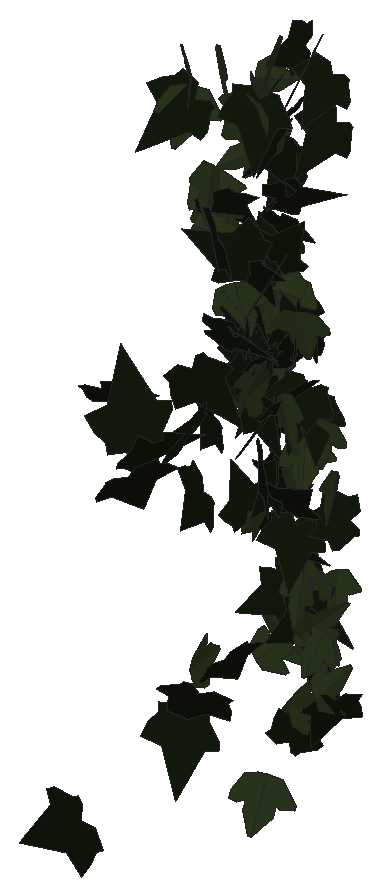
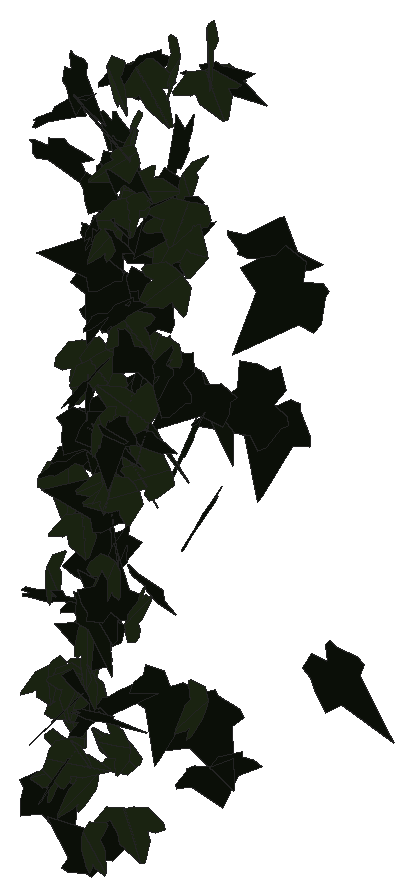
# SketchUp Ruby script. Lengths in inches.
U = 1.inch
M = Sketchup.active_model
def pt(a) = Geom::Point3d.new(a.map { |v| v * U })
def face(e, loops, mat)
  f = e.add_face(loops[0].map { |a| pt(a) })
  loops[1..].each { |l| e.add_face(l.map { |a| pt(a) }).erase! }
  f.material = f.back_material = mat if mat
  f
end
# faces: each face lists its corners as indices into pts; further lists are holes
def faces(e, pts, list, mat = nil) = list.each { |f| face(e, (f[0].is_a?(Array) ? f : [f]).map { |l| l.map { |i| pts[i] } }, mat) }
# xy, xz, yz: faces in a plane at the given z, y or x. An outline is a flat list of corners, or four numbers for a rectangle; further outlines are holes
def ring(l) = l.size == 4 ? [[l[0], l[1]], [l[2], l[1]], [l[2], l[3]], [l[0], l[3]]] : l.each_slice(2).to_a
def flat(e, list, mat, &to3) = list.each { |f| face(e, (f[0].is_a?(Array) ? f : [f]).map { |l| ring(l).map { |u, v| to3.(u, v) } }, mat) }
def xy(e, z, list, mat = nil) = flat(e, list, mat) { |x, y| [x, y, z] }
def xz(e, y, list, mat = nil) = flat(e, list, mat) { |x, z| [x, y, z] }
def yz(e, x, list, mat = nil) = flat(e, list, mat) { |y, z| [x, y, z] }
def lines(e, pts, list) = list.each { |a, b| e.add_line(pt(pts[a]), pt(pts[b])) }
# prism: a flat outline (further loops are holes) pulled along v
def prism(e, loops, v, mat = nil)
  f = face(e, loops, mat); d = Geom::Vector3d.new(v.map { |x| x * U })
  f.pushpull(f.normal.samedirection?(d) ? d.length : -d.length)
end
def box(e, o, s, mat = nil) = prism(e, [[o, [o[0] + s[0], o[1], o[2]], [o[0] + s[0], o[1] + s[1], o[2]], [o[0], o[1] + s[1], o[2]]]], [0, 0, s[2]], mat)
def at(x, y, z, deg = 0) = Geom::Transformation.translation(pt([x, y, z])) * Geom::Transformation.rotation(ORIGIN, Z_AXIS, deg.degrees)
def axes(o, x, y, z) = Geom::Transformation.new([*x, 0, *y, 0, *z, 0, *pt(o).to_a, 1])
def part(name) = M.definitions.add(name)
# library, detail: a bought-in or finely detailed component or shape, given as its bounding box
def library(name, o, s) = part(name).tap { |d| box(d.entities, o, s) }
def detail(e, o, s) = box(e.add_group.entities, o, s)
def put(e, d, t, mat = nil) = e.add_instance(d, t).tap { |i| i.material = mat if mat }
def group(e, t, mat = nil) = e.add_group.tap { |g| g.transformation = t; g.material = mat if mat }.entities
root = M.entities
M.materials.add("efeu1").color = [18, 25, 13]
M.materials.add("efeu2").color = [43, 57, 29]
c1 = part("ivyleaf_9")
p = [[1.54,2.16,1.25],[1.36,2.04,1.19],[-0.21,0.99,0.68],[-0.71,1.11,0.82],[-0.85,0.86,0.67],[-0.8,0.17,0.21],
  [-0.9,-0.01,0.1],[-0.67,-0.16,-0.02],[-0.08,-0.08,-0.05],[-0.03,-0.6,-0.4],[0.65,-0.88,-0.66],[0.83,-0.6,-0.49],
  [1.29,-0.42,-0.43],[1.8125,-0.07,-0.26],[1.21,0.44,0.15]]
faces(c1.entities,p,[[0,1,2,3,4,5,6,7,8,9,10,11,12,13,14]],"efeu1")
c2 = part("ivyleaf_10")
p = [[0,0.5,-0.03],[-0.0625,2.02,-0.43],[-0.19,2.01,-0.46],[-0.54,1.05,-0.29],[-0.52,0.625,-0.18],[-0.83,0.76,-0.28],
  [-1.16,0.64,-0.33],[-1.15,0.33,-0.24],[-0.77,-0.39,0.02],[-0.3,-0.51,0.16],[0.04,-0.48,0.23],[-0.02,2.01,-0.4375],
  [-0.06,2.01,-0.43],[0.04,-0.49,0.23],[0.67,-0.49,0.14],[1.38,0.36,-0.2],[1.375,0.51,-0.24],[0.81,0.65,-0.19],
  [0.62,0.59,-0.15],[0.6,1.09,-0.28],[0.5,1.23,-0.31]]
faces(c2.entities,p,[[0,1,2,3,4,5,6,7,8,9,10],[11,12,0,13,14,15,16,17,18,19,20]],"efeu2")
put(root,c1,axes([507.44,115.02,209.63],[0.08997,-0.01027,-1.35378],[-1.25282,-0.59245,-0.07234],[-0.63793,1.16206,-0.04885]))
put(root,c1,axes([508.96,117.2,228.68],[-1.34114,-0.18158,0.15582],[0.16312,0.00251,1.30505],[-0.19503,1.2508,0.02]))
put(root,c1,axes([506.04,118.68,229.07],[1.25105,0.55078,0.11177],[0.01308,0.22191,-1.31853],[-0.60591,1.142,0.20231]))
put(root,c1,axes([506.1,120.25,223.99],[0.4219,1.17908,-0.04223],[-0.01786,-0.0373,-1.29179],[-1.27404,0.39097,0.00412]))
put(root,c1,axes([505.62,121.05,224.76],[0.5397,0.46317,1.00584],[0.78935,0.63368,-0.70835],[-0.84746,0.88519,-0.01921]))
put(root,c1,axes([508.71,123.16,235.53],[0.12597,-0.53017,1.05207],[0.21043,-0.99273,-0.56445],[1.2154,0.22683,-0.01132]))
put(root,c1,axes([507.36,122.56,225.4],[-0.38072,1.00645,0.44945],[-0.22304,0.38477,-1.10713],[-1.16171,-0.40371,0.06527]))
put(root,c1,axes([506.3,124.34,241.09],[-1.0487,-0.46693,0.20114],[-0.15215,-0.15224,-1.11784],[0.5242,-0.97832,0.07795]))
put(root,c1,axes([505.75,124.66,209.75],[-0.47823,-1.02183,-0.19653],[0.05573,0.18354,-1.1579],[1.12091,-0.44508,-0.02628]))
put(root,c1,axes([506.83,124.12,211.76],[0.2588,0.74456,-0.84826],[-0.66024,-0.60564,-0.76177],[-0.9933,0.59656,0.28533]))
put(root,c2,axes([506.02,124.44,241.03],[0.87954,0.69197,-0.27208],[-0.21436,-0.17045,-1.11142],[-0.76967,0.83823,-0.00139]))
put(root,c1,axes([505.96,125.45,220.92],[-0.08084,-0.67951,0.85136],[-0.06969,-0.81623,-0.71076],[1.14689,-0.09749,0.01682]))
put(root,c2,axes([506.28,124.08,242.47],[0.41246,-0.38741,-0.98564],[-0.40224,0.88964,-0.53431],[1.03001,0.50257,0.18603]))
put(root,c2,axes([506.31,125.57,236.73],[-0.01653,-0.79261,0.64627],[0.55281,-0.54136,-0.70502],[0.9368,0.30548,0.42744]))
put(root,c1,axes([505.97,124.94,227.1875],[-0.18311,-0.32095,-1.01861],[0.50476,0.86074,-0.37748],[0.99211,-0.49716,0.00405]))
put(root,c1,axes([509.87,124.8,223.77],[0.33491,-0.07966,-1.14204],[-1.15928,0.23192,-0.33275],[0.26453,1.11724,-0.01235]))
put(root,c1,axes([506.06,126.04,224.5],[0.01792,-0.5786,0.86533],[0.03632,-0.83139,-0.60196],[1.09393,0.03708,0.00581]))
put(root,c1,axes([508.85,125.83,241.18],[-0.33776,-1.00359,-0.16345],[0.06068,0.1471,-1.09319],[1.09541,-0.3176,0.01016]))
put(root,c2,axes([508.54,125.55,240.79],[0.95987,-0.02679,-0.65752],[-0.65396,0.2806,-0.89763],[0.1985,1.05399,0.22226]))
put(root,c1,axes([507.81,126.17,232.83],[-0.03618,0.02535,1.09537],[-1.0952,-0.28653,-0.02637],[0.30855,-1.01407,0.03484]))
put(root,c2,axes([506.14,124.98,212.54],[0.01911,-0.0001,1.0335],[-0.43086,0.9103,0.00748],[-0.98297,-0.39901,0.01681]))
put(root,c2,axes([506.44,126.13,242.39],[-0.44859,0.65457,-0.70694],[0.37319,-0.58561,-0.80606],[-0.94839,-0.54005,0.0172]))
put(root,c2,axes([508.87,126.05,207.02],[1.0544,0.46078,-0.17471],[-0.17122,-0.05763,-1.12264],[-0.50125,0.98896,0.01598]))
put(root,c1,axes([507.33,125.39,213.08],[0.21982,1.0348,0.13224],[0.03533,0.12316,-1.09678],[-1.12544,0.20598,-0.0086]))
put(root,c1,axes([506.67,125.5,235.77],[0.86317,0.60789,0.11341],[0.08365,0.07827,-1.04418],[-0.66173,0.80283,0.01593]))
put(root,c2,axes([505.88,125.79,233.96],[-0.18129,-0.19362,-0.93562],[0.93953,0.26479,-0.22808],[0.32406,-0.87601,0.13786]))
put(root,c2,axes([506.23,126.15,234.88],[-0.93752,-0.3321,-0.36595],[0.34974,0.13822,-0.96652],[0.38825,-0.92643,-0.01302]))
put(root,c2,axes([505.82,126.24,235.84],[0.70934,0.69682,0.28521],[0.18068,0.21902,-0.99546],[-0.78831,0.67721,0.02848]))
put(root,c1,axes([509.09,126.6875,238.78],[-0.71579,0.80943,-0.05822],[0.04619,-0.03733,-1.08796],[-0.87506,-0.66408,-0.00981]))
put(root,c1,axes([505.65,126.8,228.3],[0.84135,-0.1688,0.59998],[0.61407,-0.09942,-0.82876],[0.21059,0.96427,0.01958]))
put(root,c1,axes([508.46,127.58,225.33],[-0.73678,0.42455,-0.66813],[0.42124,-0.54953,-0.80843],[-0.71707,-0.75904,0.21158]))
put(root,c2,axes([505.71,127.2,233.07],[-0.76525,-0.01167,-0.63167],[0.65559,-0.04987,-0.73549],[-0.0255,-0.93192,0.04727]))
put(root,c2,axes([507.19,127.71,226.29],[0.13801,-0.90063,0.35682],[0.02235,-0.34345,-0.94565],[1.04063,0.12682,-0.02701]))
put(root,c2,axes([508.88,127.62,225.26],[-0.76283,0.4005,-0.6504],[0.42127,-0.53437,-0.81406],[-0.6825,-0.77747,0.22448]))
put(root,c2,axes([506.88,128.1,237.125],[-0.19217,-0.08229,0.95261],[-0.22671,-0.9047,-0.12693],[0.96701,-0.22846,0.15955]))
put(root,c1,axes([506.95,127.05,231.89],[1.0143,0.44026,-0.21916],[-0.21302,-0.07567,-1.07862],[-0.48218,0.95954,0.0155]))
put(root,c2,axes([506.32,127.36,230.08],[0.89877,0.3439,0.34767],[0.26468,0.27058,-0.92396],[-0.44524,0.85504,0.15256]))
put(root,c2,axes([507.61,127.02,225.68],[0.13359,0.025,1.04989],[-0.49921,0.90565,0.03557],[-0.96964,-0.46282,0.12633]))
put(root,c1,axes([506.86,127.71,226.78],[-0.91082,0.6213,0.08213],[-0.06815,0.04749,-1.0894],[-0.67296,-0.84571,-0.00084]))
put(root,c1,axes([505.74,127.71,229.44],[0.97194,-0.39811,-0.01221],[-0.00942,0.0093,-1.02342],[0.43004,0.89998,0.00518]))
put(root,c1,axes([507.88,128.03,231.24],[-0.68619,0.60856,-0.55886],[0.36228,-0.4246,-0.91258],[-0.79846,-0.71565,0.06621]))
put(root,c1,axes([506.02,127.82,228.96],[0.67776,-0.69422,-0.18064],[0.03874,0.26125,-0.95113],[0.7719,0.59644,0.20635]))
put(root,c1,axes([507.35,128.84,220.66],[0.11805,-0.25377,-0.92422],[0.6525,-0.65756,0.27257],[-0.75533,-0.60771,0.09102]))
put(root,c2,axes([509.03,128.38,216.18],[0.9726,-0.36527,0.1887],[0.18449,-0.06158,-1.01066],[0.39998,0.91658,0.0073]))
put(root,c2,axes([507.68,128.48,242.33],[0.44859,-0.80434,0.22061],[0.0845,-0.19827,-0.94121],[0.8944,0.42215,-0.02172]))
put(root,c1,axes([508.1,128.42,219.93],[0.9963,0.16764,-0.22796],[0.23199,0.04388,0.9751],[0.18709,-0.94717,0.00483]))
put(root,c1,axes([506.52,127.92,219.23],[-0.84481,0.10836,-0.41463],[-0.42477,0.06608,0.82122],[0.13663,0.87549,-0.01066]))
put(root,c1,axes([508.7,127.79,225.5],[0.07501,1.0197,0.12341],[-0.04429,0.12159,-1.06173],[-1.10782,0.06418,0.05081]))
put(root,c1,axes([506.59,128.35,224.45],[0.46268,-0.77355,-0.44589],[-0.22098,0.37678,-0.91963],[0.92926,0.47475,0.00332]))
put(root,c2,axes([507.21,127.91,239.12],[-0.45445,0.66627,0.7094],[-0.44787,0.5435,-0.81817],[-0.92731,-0.58902,0.0475]))
put(root,c1,axes([507.01,128.71,225.55],[-0.97848,0.22479,-0.43446],[0.43938,-0.09503,-0.97079],[-0.26352,-0.99314,-0.00545]))
put(root,c1,axes([507.68,128.39,227.42],[-0.76916,0.71124,-0.03933],[0.0289,-0.02672,-1.04678],[-0.76868,-0.71269,-0.00001]))
put(root,c1,axes([506.18,128.85,226.64],[-0.91785,-0.30376,-0.2525],[0.25534,0.05967,-0.93832],[0.33344,-0.88184,0.02349]))
put(root,c1,axes([506.66,128.03,228.79],[0.28397,-0.16805,-0.94821],[-0.81398,0.51313,-0.32441],[0.58307,0.79819,0.00892]))
put(root,c1,axes([506.85,127.7,226.29],[0.45607,0.49532,0.79481],[0.35402,0.70327,-0.66241],[-0.91765,0.51749,0.13946]))
put(root,c2,axes([507.16,127.86,239.62],[0.1305,0.07209,-1.06108],[-0.38997,0.96423,0.02638],[1.03352,0.35472,0.14394]))
put(root,c1,axes([508.37,129,218.44],[-0.45789,-0.83346,-0.21433],[0.15488,0.15787,-0.97082],[0.91422,-0.44419,0.05712]))
put(root,c2,axes([506.05,129.31,218.43],[-0.155,-0.02636,0.99927],[0.49477,-0.85593,0.04674],[0.91261,0.45956,0.14438]))
put(root,c2,axes([508.96,128.5625,229.17],[-1.0021,-0.3163,-0.06562],[0.07047,0.00409,-1.01935],[0.34113,-0.93,0.01784]))
put(root,c1,axes([508.83,129.17,225.34],[-0.51747,-0.86558,-0.0449],[0.02622,0.0359,-1.02891],[0.93562,-0.47973,0.004]))
put(root,c1,axes([505.81,129.24,226.01],[-0.21173,0.05111,0.8772],[-0.09857,-0.86208,0.03227],[0.90727,-0.08174,0.20822]))
put(root,c1,axes([507.35,128.89,231.55],[-0.437,-0.09411,0.84024],[0.81337,-0.38421,0.34572],[0.33183,0.81783,0.25911]))
put(root,c2,axes([509.58,128.99,213.24],[0.9711,-0.11072,-0.22862],[-0.22949,0.07106,-0.94112],[0.13418,0.92292,0.04504]))
put(root,c1,axes([509.14,129.23,242.3],[-0.64052,0.47663,-0.63476],[0.48774,-0.41164,-0.7907],[-0.67941,-0.74486,0.03079]))
put(root,c2,axes([506.67,128.9,211.65],[0.59089,0.00255,-0.68115],[0.7065,0.03982,0.56849],[0.03477,-0.85248,0.02452]))
put(root,c1,axes([509.14,129.5,224.7],[-0.21326,-0.93064,-0.05289],[0.13034,0.02601,-0.98247],[0.99812,-0.20224,0.117]))
put(root,c2,axes([507.57,129.55,229.56],[0.24724,0.30911,0.94114],[-0.55467,-0.74519,0.39984],[0.8712,-0.56216,-0.01252]))
put(root,c2,axes([505.38,128.6,225.08],[0.28419,0.25641,0.99116],[0.64866,0.74106,-0.37982],[-0.84579,0.65449,0.04174]))
put(root,c2,axes([506.21,129.375,231.81],[0.43438,0.61703,-0.47359],[-0.31367,-0.35335,-0.76471],[-0.76653,0.49425,0.04454]))
put(root,c2,axes([509.54,129.16,223.79],[-1.04599,-0.16051,0.06807],[-0.04444,-0.14796,-1.01072],[0.18185,-0.95938,0.14449]))
put(root,c1,axes([507.67,129.84,235.69],[-0.21757,-0.07069,0.89172],[-0.37315,-0.79984,-0.153],[0.85094,-0.36881,0.1609]))
put(root,c1,axes([508.15,129.95,213.35],[-0.26613,-0.45234,0.77032],[-0.35548,-0.66374,-0.53545],[0.8673,-0.41085,0.01691]))
put(root,c1,axes([507.03,129.88,214.32],[-0.48449,-0.36942,0.66604],[-0.40699,-0.53023,-0.59262],[0.68697,-0.57467,0.11863]))
put(root,c1,axes([509.91,129.67,238.81],[-0.98814,-0.32416,-0.09378],[0.08423,0.04982,-1.00927],[0.35349,-0.91803,-0.02165]))
put(root,c1,axes([507.85,129.88,228.7],[-0.06546,-0.0725,-0.91372],[0.85551,-0.39096,-0.02328],[-0.41783,-0.78913,0.09548]))
put(root,c1,axes([507.45,129.0625,233.5],[0.88337,0.27108,-0.42302],[-0.42251,-0.11234,-0.89602],[-0.31651,0.90656,0.01546]))
put(root,c1,axes([506.78,129.82,232.4],[-0.26718,-0.85675,-0.04992],[0.01475,0.04602,-0.92742],[0.92662,-0.24776,0.00037]))
put(root,c2,axes([509.18,129.02,213.59],[-0.15302,-0.66704,0.7175],[0.32919,0.62999,0.69858],[-0.98274,0.31489,0.12228]))
put(root,c1,axes([506.91,129.125,218.16],[0.30495,0.81151,0.05275],[-0.06369,-0.03311,0.89239],[0.87583,-0.28496,0.04653]))
put(root,c2,axes([508.8,128.6875,209.79],[-0.04756,0.30369,0.94823],[-0.20139,0.89267,-0.31859],[-1.01816,-0.19075,0.01872]))
put(root,c1,axes([509.39,130.1,240.8],[-0.45861,-0.79483,0.31397],[-0.03743,-0.32099,-0.9296],[0.91748,-0.41039,0.11901]))
put(root,c1,axes([506.58,129.82,222.36],[-0.2177,-0.01119,-0.86816],[0.87531,-0.20864,-0.20063],[-0.2163,-0.83304,0.06191]))
put(root,c2,axes([508.4375,129.5,222.22],[0.60676,0.7835,-0.10498],[-0.0709,-0.07714,-1.00263],[-0.85022,0.56557,0.00869]))
put(root,c1,axes([506.63,129.74,239.61],[-0.60846,0.4749,-0.53114],[0.29358,-0.45508,-0.75195],[-0.69361,-0.60921,0.14766]))
put(root,c1,axes([506.91,129.24,223.5],[0.57039,-0.00069,0.85573],[0.88854,0.01527,-0.54918],[-0.01348,0.97761,0.00918]))
put(root,c2,axes([505.78,129.29,227.84],[-0.38935,-0.49947,0.74746],[0.54986,0.51257,0.63605],[-0.76885,0.6195,0.07637]))
put(root,c1,axes([507,129.74,217.11],[0.52596,-0.36535,0.72951],[0.65774,-0.35233,-0.63059],[0.54496,0.77786,0.05702]))
put(root,c2,axes([507.52,129.84,229.76],[0.55642,0.61614,-0.44637],[-0.31863,-0.31255,-0.83494],[-0.74574,0.59326,0.02369]))
put(root,c1,axes([507.23,129.17,234.41],[0.58389,0.03059,0.8374],[0.83379,0.25803,-0.54929],[-0.24923,0.9349,0.12421]))
put(root,c1,axes([507.95,129.78,227.3],[-0.08656,0.71042,-0.69149],[-0.0665,-0.66951,-0.73624],[-1.04876,-0.01618,0.10376]))
put(root,c2,axes([506.84,129.02,224.7],[-0.12367,-0.14055,-1.01184],[0.57205,0.81633,-0.18748],[0.89437,-0.54157,-0.02]))
put(root,c1,axes([505.55,129.86,231.3],[-0.37499,-0.19576,-0.84752],[0.82136,0.29707,-0.41121],[0.38036,-0.8345,0.05242]))
put(root,c1,axes([507.14,130.08,236.03],[-0.84981,-0.23007,-0.29311],[0.28533,0.10035,-0.85232],[0.27014,-0.82977,-0.0218]))
put(root,c1,axes([509.82,129.82,209.91],[0.118,0.70996,-0.62949],[-0.06806,-0.60241,-0.74669],[-1.00529,0.12412,-0.02334]))
put(root,c2,axes([505.88,129.86,237.71],[0.46849,0.76292,-0.13977],[-0.06405,-0.12088,-0.91269],[-0.83418,0.43775,-0.00842]))
put(root,c2,axes([506.05,130.02,213],[-0.27668,0.18619,-0.78814],[0.69156,-0.40574,-0.3288],[-0.48172,-0.68943,-0.01935]))
put(root,c1,axes([507.65,130.12,229.16],[0.2997,-0.89627,-0.13812],[-0.04466,0.12622,-0.97577],[0.97752,0.28056,-0.00224]))
put(root,c1,axes([507.23,130.08,238.39],[-0.46987,0.64626,-0.40986],[0.17915,-0.3621,-0.808],[-0.79763,-0.46203,0.05996]))
put(root,c1,axes([510,130.48,218.75],[-0.88556,0.07357,0.49753],[-0.50938,-0.33282,-0.78751],[0.11741,-0.88906,0.33598]))
put(root,c2,axes([508.71,130.2,212.21],[0.99033,-0.12574,0.11104],[0.11279,-0.02425,-0.96253],[0.1379,0.92285,-0.01016]))
put(root,c1,axes([507.5,129.75,207.29],[-0.18222,-0.09636,0.90838],[0.93043,0.15717,0.19111],[-0.18706,0.8756,0.06567]))
put(root,c2,axes([507.77,129.9375,217.33],[-0.04266,-0.88871,-0.36018],[-0.01855,0.34723,-0.92464],[1.02995,-0.03056,-0.03157]))
put(root,c2,axes([507.55,130.34,215.77],[-0.70092,0.25941,-0.53053],[0.37626,-0.43281,-0.68987],[-0.49035,-0.70292,0.22899]))
put(root,c2,axes([509.47,129.41,210.48],[0.20852,0.15544,-0.9551],[0.27192,0.89426,0.21247],[0.96849,-0.28455,0.14599]))
put(root,c1,axes([506.92,130.41,227.17],[-0.89306,-0.04708,0.07482],[-0.0768,-0.01651,-0.86128],[0.05219,-0.82987,0.01289]))
put(root,c2,axes([506.58,130.5625,227.68],[-0.00445,-0.85702,0.44016],[0.347,-0.41205,-0.79878],[0.89879,0.15484,0.31057]))
put(root,c2,axes([508.03,130.07,215.18],[0.82627,0.46313,0.29792],[0.21809,0.21749,-0.92659],[-0.5462,0.78746,0.0807]))
put(root,c1,axes([508.57,130.22,211.5625],[0.51292,-0.72552,-0.32468],[-0.18299,0.26222,-0.90183],[0.83317,0.50424,0.00181]))
put(root,c1,axes([508.51,129.87,214.3],[-0.94843,0.28638,0.06175],[0.04007,-0.0773,0.95849],[0.31331,0.87678,0.06434]))
put(root,c2,axes([507.9375,130.1,215.38],[0.96824,0.12293,0.26645],[0.23177,0.26293,-0.91219],[-0.20117,0.89457,0.23149]))
put(root,c2,axes([506.61,130.13,220.84],[-0.8758,0.35202,-0.15253],[0.14334,-0.06258,-0.91938],[-0.38611,-0.8217,0.00468]))
put(root,c2,axes([505.91,129.77,239.68],[0.03378,-0.30357,-0.84631],[0.51399,0.68715,-0.24756],[0.78466,-0.43704,0.1986]))
put(root,c1,axes([506.14,130.58,219.46],[0.89123,-0.10633,0.21552],[-0.22095,0.03382,0.86529],[-0.12026,-0.85016,0.00747]))
put(root,c1,axes([507.72,130.29,241.65],[-0.81887,0.44132,0.1842],[-0.16641,0.08736,-0.91239],[-0.48587,-0.77371,0.00205]))
put(root,c2,axes([508.65,130.69,211.78],[0.22732,0.11628,-0.94012],[-0.86858,-0.36025,-0.25458],[-0.37804,0.89762,0.01961]))
put(root,c2,axes([509.01,130.77,220.17],[0.20884,-0.70906,0.52201],[0.36375,-0.41909,-0.71479],[0.80184,0.37479,0.1883]))
put(root,c1,axes([508.34,130.125,214.3],[0.61277,-0.55922,-0.47978],[-0.14918,0.49169,-0.79655],[0.7686,0.54128,0.22789]))
put(root,c2,axes([505.69,130.12,224.66],[-0.36187,-0.10975,-0.82111],[0.82812,0.18966,-0.36584],[0.23525,-0.83645,0.02479]))
put(root,c1,axes([507.53,130.01,218.76],[-0.42541,0.85345,0.10845],[-0.0204,0.10608,-0.97715],[-0.92835,-0.39342,-0.02822]))
put(root,c2,axes([507.0625,130.78,208.65],[0.22386,-0.78513,0.38766],[0.10572,-0.35968,-0.84451],[0.93268,0.22922,0.00268]))
put(root,c1,axes([506.5,130.21,227.54],[0.60712,0.41188,-0.51227],[-0.47153,-0.23483,-0.72242],[-0.50846,0.70957,0.05827]))
put(root,c2,axes([509.37,130.56,215.46],[0.22513,0.86705,-0.2323],[-0.03639,-0.22158,-0.92723],[-0.96631,0.21035,-0.0192]))
put(root,c2,axes([506.28,130.45,225.21],[-0.17327,0.8116,-0.09471],[0.01291,-0.09046,-0.86038],[-0.88194,-0.16078,0.00601]))
put(root,c2,axes([506.62,129.85,236.11],[0.10773,0.20377,0.86513],[-0.24097,0.81475,-0.17973],[-0.89303,-0.19527,0.15286]))
put(root,c1,axes([507.12,130.95,214.51],[-0.86874,-0.03065,0.29465],[-0.28018,-0.27231,-0.79666],[0.12735,-0.80818,0.25725]))
